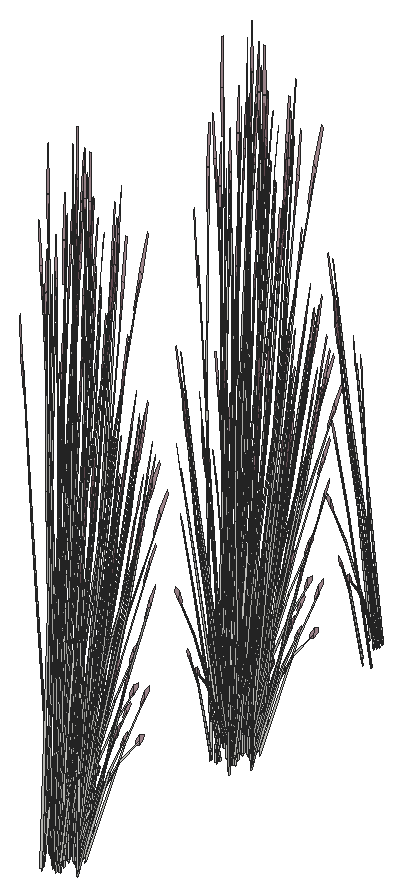
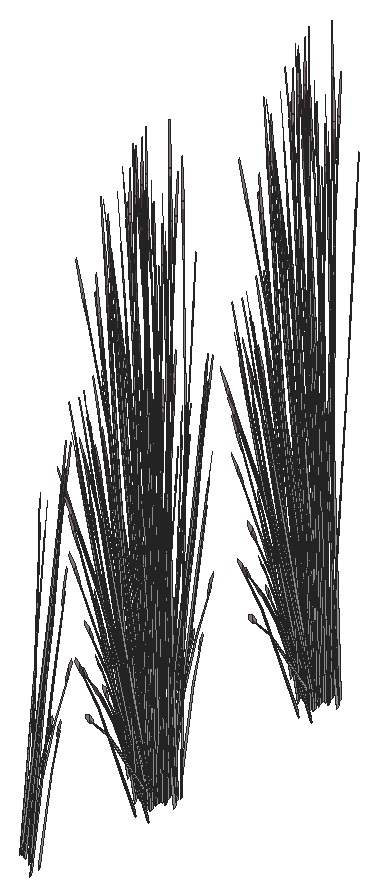
# SketchUp Ruby script. Lengths in inches.
U = 1.inch
M = Sketchup.active_model
def pt(a) = Geom::Point3d.new(a.map { |v| v * U })
def face(e, loops, mat)
  f = e.add_face(loops[0].map { |a| pt(a) })
  loops[1..].each { |l| e.add_face(l.map { |a| pt(a) }).erase! }
  f.material = f.back_material = mat if mat
  f
end
# faces: each face lists its corners as indices into pts; further lists are holes
def faces(e, pts, list, mat = nil) = list.each { |f| face(e, (f[0].is_a?(Array) ? f : [f]).map { |l| l.map { |i| pts[i] } }, mat) }
# xy, xz, yz: faces in a plane at the given z, y or x. An outline is a flat list of corners, or four numbers for a rectangle; further outlines are holes
def ring(l) = l.size == 4 ? [[l[0], l[1]], [l[2], l[1]], [l[2], l[3]], [l[0], l[3]]] : l.each_slice(2).to_a
def flat(e, list, mat, &to3) = list.each { |f| face(e, (f[0].is_a?(Array) ? f : [f]).map { |l| ring(l).map { |u, v| to3.(u, v) } }, mat) }
def xy(e, z, list, mat = nil) = flat(e, list, mat) { |x, y| [x, y, z] }
def xz(e, y, list, mat = nil) = flat(e, list, mat) { |x, z| [x, y, z] }
def yz(e, x, list, mat = nil) = flat(e, list, mat) { |y, z| [x, y, z] }
def lines(e, pts, list) = list.each { |a, b| e.add_line(pt(pts[a]), pt(pts[b])) }
# prism: a flat outline (further loops are holes) pulled along v
def prism(e, loops, v, mat = nil)
  f = face(e, loops, mat); d = Geom::Vector3d.new(v.map { |x| x * U })
  f.pushpull(f.normal.samedirection?(d) ? d.length : -d.length)
end
def box(e, o, s, mat = nil) = prism(e, [[o, [o[0] + s[0], o[1], o[2]], [o[0] + s[0], o[1] + s[1], o[2]], [o[0], o[1] + s[1], o[2]]]], [0, 0, s[2]], mat)
def at(x, y, z, deg = 0) = Geom::Transformation.translation(pt([x, y, z])) * Geom::Transformation.rotation(ORIGIN, Z_AXIS, deg.degrees)
def axes(o, x, y, z) = Geom::Transformation.new([*x, 0, *y, 0, *z, 0, *pt(o).to_a, 1])
def part(name) = M.definitions.add(name)
# library, detail: a bought-in or finely detailed component or shape, given as its bounding box
def library(name, o, s) = part(name).tap { |d| box(d.entities, o, s) }
def detail(e, o, s) = box(e.add_group.entities, o, s)
def put(e, d, t, mat = nil) = e.add_instance(d, t).tap { |i| i.material = mat if mat }
def group(e, t, mat = nil) = e.add_group.tap { |g| g.transformation = t; g.material = mat if mat }.entities
root = M.entities
M.materials.add("LightPink_Translucent").color = [144, 107, 117]
M.materials["LightPink_Translucent"].alpha = 0.75
c1 = part("blade")
p = [[2.15,0.21,22],[0,0.17,0],[0.09,0.45,0],[2.18,0.31,22],[2.29,0.31,22],[0.38,0.45,0],
  [2.48,0.24,33],[2.49,0.24,33],[2.48,0.22,33]]
faces(c1.entities,p,[[0,1,2,3],[4,5,2,3],[6,3,4,7],[8,0,3,6]])
c2 = part("seeds")
p = [[0.3,-0.1,1.38],[-0.01,-0.03,1.59],[-0.01,-0.03,0.03],[0.14,-0.07,-0.07],[0.29,-0.03,3],[0.15,0.01,3.11]]
faces(c2.entities,p,[[0,1,2,3],[1,0,4,5]],"LightPink_Translucent")
c3 = part("blade with seeds")
put(c3.entities,c1,at(0,0,0))
put(c3.entities,c2,axes([2.4,0.25,30.99],[1.5799,-0.05474,1.17369],[-0.12525,1.92788,0.29478],[-0.07173,-0.02425,1.56792]))
put(root,c3,axes([330.71,560.5,1400.21],[0.17124,-0.42022,-0.44739],[0.35581,0.20224,0.21531],[0,-0.09687,1.43643]))
put(root,c3,axes([330.71,582.22,1400.21],[0.17124,-0.42022,-0.44739],[0.35581,0.20224,0.21531],[0,-0.09687,1.43643]))
put(root,c3,axes([331.15,561.85,1400.2],[-0.11516,-0.40207,0],[0.32884,-0.1408,0],[0,0,1.54371]))
put(root,c3,axes([331.15,583.57,1400.2],[-0.11516,-0.40207,0],[0.32884,-0.1408,0],[0,0,1.54371]))
put(root,c3,axes([330.73,562.7,1399.49],[0.05712,-0.02538,1.76342],[0.34359,0.13968,-0.26939],[0.01005,0.15742,0.30037]))
put(root,c3,axes([330.73,584.42,1399.49],[0.05712,-0.02538,1.76342],[0.34359,0.13968,-0.26939],[0.01005,0.15742,0.30037]))
put(root,c3,axes([330.8,562.84,1402.53],[-0.1064,0.35863,-0.35414],[-0.31043,-0.1046,0.4572],[0.02846,0.14439,0.87481]))
put(root,c3,axes([330.8,584.5625,1402.53],[-0.1064,0.35863,-0.35414],[-0.31043,-0.1046,0.4572],[0.02846,0.14439,0.87481]))
put(root,c3,axes([331.61,561.0625,1400.21],[-0.17124,0.42022,-0.44739],[-0.35581,-0.20224,0.21531],[0,0.09687,1.43643]))
put(root,c3,axes([331.61,582.78,1400.21],[-0.17124,0.42022,-0.44739],[-0.35581,-0.20224,0.21531],[0,0.09687,1.43643]))
put(root,c3,axes([331.43,580.4,1402.73],[0.26007,-0.1585,0.0643],[0.12729,0.28902,0.50621],[-0.02512,-0.1274,0.77189]))
put(root,c3,axes([330.58,563.48,1402.72],[0.04474,0.0751,1.74944],[0.36104,0.0295,-0.27667],[0.03631,0.16562,0.14031]))
put(root,c3,axes([330.58,585.2,1402.72],[0.04474,0.0751,1.74944],[0.36104,0.0295,-0.27667],[0.03631,0.16562,0.14031]))
put(root,c3,axes([332.29,560.81,1400.47],[-0.2773,-0.3397,0.17642],[0.27945,-0.32949,0.35086],[-0.03063,0.06937,1.60407]))
put(root,c3,axes([332.29,582.52,1400.47],[-0.2773,-0.3397,0.17642],[0.27945,-0.32949,0.35086],[-0.03063,0.06937,1.60407]))
put(root,c3,axes([331.33,560.61,1400.21],[0,-0.53961,0],[0.44133,0,0],[0,0,1.79456]))
put(root,c3,axes([331.33,582.33,1400.21],[0,-0.53961,0],[0.44133,0,0],[0,0,1.79456]))
put(root,c3,axes([331.34,580.43,1402.73],[0.34777,0.12192,0.48003],[-0.11892,0.40083,0.3958],[-0.0209,-0.15763,0.9933]))
put(root,c3,axes([331.34,599.35,1402.73],[0.34777,0.12192,0.48003],[-0.11892,0.40083,0.3958],[-0.0209,-0.15763,0.9933]))
put(root,c3,axes([330.92,560.71,1400.43],[0.39767,0.22603,0.24065],[-0.19139,0.46966,0.50002],[0,-0.10827,1.60543]))
put(root,c3,axes([330.92,582.43,1400.43],[0.39767,0.22603,0.24065],[-0.19139,0.46966,0.50002],[0,-0.10827,1.60543]))
put(root,c3,axes([331.55,560.82,1400.29],[0,0.53934,-0.05637],[-0.44133,0,0],[0,0.01695,1.79368]))
put(root,c3,axes([331.55,582.54,1400.29],[0,0.53934,-0.05637],[-0.44133,0,0],[0,0.01695,1.79368]))
put(root,c3,axes([330.79,560.39,1400.72],[-0.38326,0.02879,0.44739],[-0.03466,-0.47788,-0.21531],[0.06861,-0.04843,1.43643]))
put(root,c3,axes([330.79,582.11,1400.72],[-0.38326,0.02879,0.44739],[-0.03466,-0.47788,-0.21531],[0.06861,-0.04843,1.43643]))
put(root,c3,axes([330.77,562.47,1403.05],[0.1064,-0.35863,0.35414],[0.31043,0.1046,-0.4572],[0.02846,0.14439,0.87481]))
put(root,c3,axes([330.77,584.18,1403.05],[0.1064,-0.35863,0.35414],[0.31043,0.1046,-0.4572],[0.02846,0.14439,0.87481]))
put(root,c3,axes([330.61,559.57,1400.47],[-0.10196,0.46348,0.17642],[-0.3731,-0.13116,0.35086],[0.06445,-0.00226,1.60407]))
put(root,c3,axes([330.61,581.29,1400.47],[-0.10196,0.46348,0.17642],[-0.3731,-0.13116,0.35086],[0.06445,-0.00226,1.60407]))
put(root,c3,axes([331.34,561.87,1400.29],[0.15345,0.53576,-0.06012],[-0.43845,0.18773,0],[0.00536,0.01871,1.72173]))
put(root,c3,axes([331.34,583.59,1400.29],[0.15345,0.53576,-0.06012],[-0.43845,0.18773,0],[0.00536,0.01871,1.72173]))
put(root,c3,axes([330.43,580.72,1400.375],[-0.22066,-0.46731,0],[0.36918,-0.26061,-0.51607],[0.08408,-0.05936,1.63711]))
put(root,c3,axes([330.84,562.52,1402.98],[0.16845,0.3792,-0.71045],[-0.34676,0.21133,0.08574],[0.03939,0.18322,1.00501]))
put(root,c3,axes([330.84,584.24,1402.98],[0.16845,0.3792,-0.71045],[-0.34676,0.21133,0.08574],[0.03939,0.18322,1.00501]))
put(root,c3,axes([332.61,561.17,1400.2],[-0.44111,-0.00373,-0.04976],[0,-0.52122,0.49943],[-0.01386,0.11865,1.58352]))
put(root,c3,axes([332.61,582.88,1400.2],[-0.44111,-0.00373,-0.04976],[0,-0.52122,0.49943],[-0.01386,0.11865,1.58352]))
put(root,c3,axes([331.74,559.6,1400.47],[-0.37926,0.12378,0.17642],[-0.09365,-0.46065,0.35086],[0.03382,0.06712,1.60407]))
put(root,c3,axes([331.74,581.32,1400.47],[-0.37926,0.12378,0.17642],[-0.09365,-0.46065,0.35086],[0.03382,0.06712,1.60407]))
put(root,c3,axes([331.35,579.59,1400.77],[0.04528,0.27194,1.1486],[-0.25117,-0.15062,0.84392],[0.02703,-0.13924,0.25299]))
put(root,c3,axes([331.35,598.51,1400.77],[0.04528,0.27194,1.1486],[-0.25117,-0.15062,0.84392],[0.02703,-0.13924,0.25299]))
put(root,c3,axes([331.1875,563.75,1403.65],[0.2439,-0.26754,-0.06488],[0.22348,0.29302,-0.29416],[0.01573,0.08303,0.97024]))
put(root,c3,axes([331.1875,585.46,1403.65],[0.2439,-0.26754,-0.06488],[0.22348,0.29302,-0.29416],[0.01573,0.08303,0.97024]))
put(root,c3,axes([331.12,560.27,1400.36],[-0.29264,0.42323,0.45755],[-0.34767,-0.3736,0.17955],[0.07055,-0.04224,1.58856]))
put(root,c3,axes([331.12,581.99,1400.36],[-0.29264,0.42323,0.45755],[-0.34767,-0.3736,0.17955],[0.07055,-0.04224,1.58856]))
put(root,c3,axes([331.62,560.9375,1400.21],[0.24637,0.30123,0],[-0.24637,0.30123,0],[0,0,1.69266]))
put(root,c3,axes([331.62,582.65,1400.21],[0.24637,0.30123,0],[-0.24637,0.30123,0],[0,0,1.69266]))
put(root,c3,axes([331.62,560.58,1400.72],[0.17124,-0.42022,0.44739],[0.35581,0.20224,-0.21531],[0,0.09687,1.43643]))
put(root,c3,axes([331.62,582.3,1400.72],[0.17124,-0.42022,0.44739],[0.35581,0.20224,-0.21531],[0,0.09687,1.43643]))
put(root,c3,axes([331.47,562.04,1400.2],[0.35581,0.20937,0],[-0.17124,0.43505,0],[0,0,1.74954]))
put(root,c3,axes([331.47,583.76,1400.2],[0.35581,0.20937,0],[-0.17124,0.43505,0],[0,0,1.74954]))
put(root,c3,axes([330.96,562.6,1402.68],[0.34695,0.11691,-0.51099],[-0.11892,0.40083,-0.3958],[0.03181,0.16138,0.97773]))
put(root,c3,axes([330.96,584.32,1402.68],[0.34695,0.11691,-0.51099],[-0.11892,0.40083,-0.3958],[0.03181,0.16138,0.97773]))
put(root,c3,axes([330.67,562.62,1403.03],[0.34538,-0.21713,-0.1216],[0.16972,0.38536,-0.67495],[0.04557,0.16239,1.02557]))
put(root,c3,axes([330.67,584.34,1403.03],[0.34538,-0.21713,-0.1216],[0.16972,0.38536,-0.67495],[0.04557,0.16239,1.02557]))
put(root,c3,axes([331.5,560.48,1400.38],[-0.44609,-0.09826,0.49198],[0.09078,-0.55493,0.19306],[0.06519,0.05359,1.70813]))
put(root,c3,axes([331.5,582.2,1400.38],[-0.44609,-0.09826,0.49198],[0.09078,-0.55493,0.19306],[0.06519,0.05359,1.70813]))
put(root,c3,axes([332.43,580.03,1402.71],[-0.03584,0.03562,1.77383],[-0.35118,-0.12018,-0.16761],[-0.01271,-0.15545,0.31391]))
put(root,c3,axes([332.43,598.95,1402.71],[-0.03584,0.03562,1.77383],[-0.35118,-0.12018,-0.16761],[-0.01271,-0.15545,0.31391]))
put(root,c3,axes([332.15,581.0625,1403.03],[-0.3879,-0.02311,-0.1216],[0.0106,-0.43749,-0.67495],[0.02694,-0.1685,1.02557]))
put(root,c3,axes([332.15,599.98,1403.03],[-0.3879,-0.02311,-0.1216],[0.0106,-0.43749,-0.67495],[0.02694,-0.1685,1.02557]))
put(root,c3,axes([332.52,561.24,1400.03],[-0.24637,0.29097,-0.30978],[-0.24637,-0.29097,0.30978],[0,0.09372,1.38974]))
put(root,c3,axes([332.52,582.96,1400.03],[-0.24637,0.29097,-0.30978],[-0.24637,-0.29097,0.30978],[0,0.09372,1.38974]))
put(root,c3,axes([331.8125,561.1875,1400.09],[0.12941,0.42699,-0.69212],[-0.37279,0.15378,-0.18165],[0.0143,0.14459,1.52773]))
put(root,c3,axes([331.8125,582.91,1400.09],[0.12941,0.42699,-0.69212],[-0.37279,0.15378,-0.18165],[0.0143,0.14459,1.52773]))
put(root,c3,axes([331.63,560.73,1400.21],[0.39487,0,0],[0,0.48281,0],[0,0,1.78407]))
put(root,c3,axes([331.63,582.45,1400.21],[0.39487,0,0],[0,0.48281,0],[0,0,1.78407]))
put(root,c3,axes([332,581.13,1403.05],[-0.23881,0.24554,0.35414],[-0.22606,-0.28036,-0.4572],[0.0344,-0.14245,0.87481]))
put(root,c3,axes([331.25,560.2,1400.72],[-0.21202,-0.39143,0.44739],[0.32115,-0.27564,-0.21531],[0.06861,0.04843,1.43643]))
put(root,c3,axes([331.25,581.91,1400.72],[-0.21202,-0.39143,0.44739],[0.32115,-0.27564,-0.21531],[0.06861,0.04843,1.43643]))
put(root,c3,axes([330.86,560.29,1400.67],[-0.04113,-0.53214,-0.29095],[0.42835,-0.03218,-0.50002],[0.07543,-0.07088,1.59708]))
put(root,c3,axes([330.86,582.01,1400.67],[-0.04113,-0.53214,-0.29095],[0.42835,-0.03218,-0.50002],[0.07543,-0.07088,1.59708]))
put(root,c3,axes([331.77,560.68,1400.62],[0.32884,-0.136,0.1448],[0.11516,0.38837,-0.41347],[0,0.08547,1.26744]))
put(root,c3,axes([331.77,582.4,1400.62],[0.32884,-0.136,0.1448],[0.11516,0.38837,-0.41347],[0,0.08547,1.26744]))
put(root,c3,axes([331.89,580.9,1402.68],[-0.25266,-0.31335,-0.51099],[0.2669,-0.27442,-0.3958],[0.03844,-0.15921,0.97773]))
put(root,c3,axes([331.89,599.8125,1402.68],[-0.25266,-0.31335,-0.51099],[0.2669,-0.27442,-0.3958],[0.03844,-0.15921,0.97773]))
put(root,c3,axes([331.65,560.71,1400.67],[0.39748,0.22252,-0.29095],[-0.19139,0.46966,-0.50002],[0.01249,0.11531,1.59708]))
put(root,c3,axes([331.65,582.43,1400.67],[0.39748,0.22252,-0.29095],[-0.19139,0.46966,-0.50002],[0.01249,0.11531,1.59708]))
put(root,c3,axes([330.81,559.11,1400.03],[0.32928,0.11539,-0.30978],[-0.08291,0.40636,0.30978],[0.06638,-0.04686,1.38974]))
put(root,c3,axes([330.81,580.83,1400.03],[0.32928,0.11539,-0.30978],[-0.08291,0.40636,0.30978],[0.06638,-0.04686,1.38974]))
put(root,c3,axes([331.72,580.34,1400.59],[-0.10032,0.0944,1.43002],[-0.30046,-0.16522,-0.30754],[0.05569,-0.20547,0.61141]))
put(root,c3,axes([331.72,599.26,1400.59],[-0.10032,0.0944,1.43002],[-0.30046,-0.16522,-0.30754],[0.05569,-0.20547,0.61141]))
put(root,c3,axes([332.52,560.82,1400.48],[0,-0.46636,0.49651],[0.39487,0,0],[0,0.10622,1.57504]))
put(root,c3,axes([332.52,582.54,1400.48],[0,-0.46636,0.49651],[0.39487,0,0],[0,0.10622,1.57504]))
put(root,c3,axes([332.6875,561.25,1400.02],[0,0.46636,-0.49651],[-0.39487,0,0],[0,0.10622,1.57504]))
put(root,c3,axes([332.6875,582.97,1400.02],[0,0.46636,-0.49651],[-0.39487,0,0],[0,0.10622,1.57504]))
put(root,c3,axes([331.63,562.66,1402.73],[-0.35104,0.10702,0.48003],[-0.06092,-0.41983,0.3958],[0.08256,0.12373,0.9933]))
put(root,c3,axes([331.63,584.38,1402.73],[-0.35104,0.10702,0.48003],[-0.06092,-0.41983,0.3958],[0.08256,0.12373,0.9933]))
put(root,c3,axes([330.73,558.93,1400.02],[0.33032,-0.23318,-0.49651],[0.19744,0.41812,0],[0.07523,-0.05311,1.57504]))
put(root,c3,axes([330.73,580.65,1400.02],[0.33032,-0.23318,-0.49651],[0.19744,0.41812,0],[0.07523,-0.05311,1.57504]))
put(root,c3,axes([331.56,562.75,1402.73],[-0.16041,0.29625,0.0643],[-0.22843,-0.17248,0.50621],[0.07385,0.09498,0.77189]))
put(root,c3,axes([331.56,584.46,1402.73],[-0.16041,0.29625,0.0643],[-0.22843,-0.17248,0.50621],[0.07385,0.09498,0.77189]))
put(root,c3,axes([331.16,561.77,1401.875],[-0.08068,-0.14973,1.71376],[0.3728,-0.12606,0.13857],[0.08426,0.23506,0.73262]))
put(root,c3,axes([331.16,583.49,1401.875],[-0.08068,-0.14973,1.71376],[0.3728,-0.12606,0.13857],[0.08426,0.23506,0.73262]))
put(root,c3,axes([331.39,560.09,1400.62],[0.06809,-0.4162,0.1448],[0.33266,0.07225,-0.41347],[0.06054,0.04274,1.26744]))
put(root,c3,axes([331.39,581.8,1400.62],[0.06809,-0.4162,0.1448],[0.33266,0.07225,-0.41347],[0.06054,0.04274,1.26744]))
put(root,c3,axes([331.87,559.36,1400.48],[-0.33032,-0.23318,0.49651],[0.19744,-0.41812,0],[0.07523,0.05311,1.57504]))
put(root,c3,axes([331.87,581.08,1400.48],[-0.33032,-0.23318,0.49651],[0.19744,-0.41812,0],[0.07523,0.05311,1.57504]))
put(root,c3,axes([331.97,581.04,1402.98],[0.00918,-0.43138,-0.71045],[0.38672,0.02897,0.08574],[0.04081,-0.18275,1.00501]))
put(root,c3,axes([331.97,599.96,1402.98],[0.00918,-0.43138,-0.71045],[0.38672,0.02897,0.08574],[0.04081,-0.18275,1.00501]))
put(root,c3,axes([331.58,561.8,1400.18],[0.37054,-0.15823,-0.19198],[0.1302,0.45581,0.00008],[0.0409,-0.01749,1.73897]))
put(root,c3,axes([331.58,583.52,1400.18],[0.37054,-0.15823,-0.19198],[0.1302,0.45581,0.00008],[0.0409,-0.01749,1.73897]))
put(root,c3,axes([331.52,562.41,1403.05],[-0.05451,-0.37564,0.35414],[0.31161,-0.09919,-0.4572],[0.0837,0.10765,0.87481]))
put(root,c3,axes([331.52,584.125,1403.05],[-0.05451,-0.37564,0.35414],[0.31161,-0.09919,-0.4572],[0.0837,0.10765,0.87481]))
put(root,c3,axes([331.58,560.44,1400.21],[0.21202,0.39143,-0.44739],[-0.32115,0.27564,0.21531],[0.06861,0.04843,1.43643]))
put(root,c3,axes([331.58,582.16,1400.21],[0.21202,0.39143,-0.44739],[-0.32115,0.27564,0.21531],[0.06861,0.04843,1.43643]))
put(root,c3,axes([331.72,560.25,1402.47],[-0.30498,-0.24231,1.38283],[0.32203,-0.37727,0.59665],[0.0984,0.22736,1.33663]))
put(root,c3,axes([331.72,581.96,1402.47],[-0.30498,-0.24231,1.38283],[0.32203,-0.37727,0.59665],[0.0984,0.22736,1.33663]))
put(root,c3,axes([332.13,580.78,1402.53],[0.23881,-0.24554,-0.35414],[0.22606,0.28036,0.4572],[0.0344,-0.14245,0.87481]))
put(root,c3,axes([332.13,599.7,1402.53],[0.23881,-0.24554,-0.35414],[0.22606,0.28036,0.4572],[0.0344,-0.14245,0.87481]))
put(root,c3,axes([331.21,562.93,1402.71],[0.00104,-0.05646,1.77383],[0.30246,-0.2491,-0.16761],[0.10506,0.08891,0.31391]))
put(root,c3,axes([331.21,584.65,1402.71],[0.00104,-0.05646,1.77383],[0.30246,-0.2491,-0.16761],[0.10506,0.08891,0.31391]))
put(root,c3,axes([332.22,580.91,1402.73],[0.29004,0.02173,0.0643],[-0.00795,0.32812,0.50621],[0.03035,-0.12569,0.77189]))
put(root,c3,axes([332.18,562.22,1400.77],[-0.19872,-0.13409,1.1486],[0.2566,-0.13625,0.84392],[0.06921,0.11541,0.25299]))
put(root,c3,axes([332.18,583.9375,1400.77],[-0.19872,-0.13409,1.1486],[0.2566,-0.13625,0.84392],[0.06921,0.11541,0.25299]))
put(root,c3,axes([331.48,562.08,1400.59],[0.00623,-0.15459,1.43002],[0.29764,-0.17268,-0.30754],[0.09188,0.18503,0.61141]))
put(root,c3,axes([331.48,583.79,1400.59],[0.00623,-0.15459,1.43002],[0.29764,-0.17268,-0.30754],[0.09188,0.18503,0.61141]))
put(root,c3,axes([332.51,580.37,1402.72],[-0.00341,-0.09282,1.74944],[-0.28775,-0.26825,-0.27667],[0.04449,-0.16261,0.14031]))
put(root,c3,axes([332.51,599.28,1402.72],[-0.00341,-0.09282,1.74944],[-0.28775,-0.26825,-0.27667],[0.04449,-0.16261,0.14031]))
put(root,c3,axes([331.12,559.88,1400.06],[0.23773,-0.35053,-0.62353],[0.29532,0.31785,-0.16365],[0.09526,-0.08744,1.37633]))
put(root,c3,axes([331.12,581.6,1400.06],[0.23773,-0.35053,-0.62353],[0.29532,0.31785,-0.16365],[0.09526,-0.08744,1.37633]))
put(root,c3,axes([332.125,580.875,1402.73],[0.25132,0.3182,0.48003],[-0.2669,0.27442,0.3958],[0.04636,-0.14929,0.9933]))
put(root,c3,axes([332.17,559.57,1400.03],[0.08291,0.40636,-0.30978],[-0.32928,0.11539,0.30978],[0.06638,0.04686,1.38974]))
put(root,c3,axes([332.17,581.29,1400.03],[0.08291,0.40636,-0.30978],[-0.32928,0.11539,0.30978],[0.06638,0.04686,1.38974]))
put(root,c3,axes([332.78,560.9,1400.375],[0.44133,0,0],[0,0.52122,-0.51607],[0,0.11871,1.63711]))
put(root,c3,axes([332.78,582.62,1400.375],[0.44133,0,0],[0,0.52122,-0.51607],[0,0.11871,1.63711]))
put(root,c3,axes([331.36,560.22,1400.67],[0.35635,-0.30962,-0.29095],[0.23697,0.43749,-0.50002],[0.08792,0.04443,1.59708]))
put(root,c3,axes([331.36,581.94,1400.67],[0.35635,-0.30962,-0.29095],[0.23697,0.43749,-0.50002],[0.08792,0.04443,1.59708]))
put(root,c3,axes([332.22,562.83,1400.67],[-0.22633,-0.01463,1.0506],[0.14947,-0.31064,0.58006],[0.08941,0.11036,0.8241]))
put(root,c3,axes([332.22,584.55,1400.67],[-0.22633,-0.01463,1.0506],[0.14947,-0.31064,0.58006],[0.08941,0.11036,0.8241]))
put(root,c3,axes([332.42,560.17,1403.05],[-0.30722,0.06665,0.35414],[-0.08112,-0.381,-0.4572],[0.08804,-0.10234,0.87481]))
put(root,c3,axes([332.42,581.89,1403.05],[-0.30722,0.06665,0.35414],[-0.08112,-0.381,-0.4572],[0.08804,-0.10234,0.87481]))
put(root,c3,axes([331.53,580.82,1401.875],[-0.06572,0.16029,1.71376],[-0.27569,-0.33172,0.13857],[0.12437,-0.20675,0.73262]))
put(root,c3,axes([331.53,599.74,1401.875],[-0.06572,0.16029,1.71376],[-0.27569,-0.33172,0.13857],[0.12437,-0.20675,0.73262]))
put(root,c3,axes([331.49,562.6,1403.03],[0.21031,-0.39918,-0.1216],[0.30457,0.22997,-0.67495],[0.10587,0.11278,1.02557]))
put(root,c3,axes([331.49,584.32,1403.03],[0.21031,-0.39918,-0.1216],[0.30457,0.22997,-0.67495],[0.10587,0.11278,1.02557]))
put(root,c3,axes([330.46,559.95,1399.59],[-0.3474,0.18671,1.28929],[-0.11057,-0.53572,0.50096],[0.21332,0.00891,1.46642]))
put(root,c3,axes([330.46,581.66,1399.59],[-0.3474,0.18671,1.28929],[-0.11057,-0.53572,0.50096],[0.21332,0.00891,1.46642]))
put(root,c3,axes([332.58,581.92,1403.03],[-0.32648,-0.25715,-0.1216],[0.18809,-0.3724,-0.67495],[0.09224,-0.12945,1.02557]))
put(root,c3,axes([331.74,562.4,1402.68],[0.34827,-0.11086,-0.51099],[0.06092,0.41983,-0.3958],[0.09354,0.12031,0.97773]))
put(root,c3,axes([331.74,584.12,1402.68],[0.34827,-0.11086,-0.51099],[0.06092,0.41983,-0.3958],[0.09354,0.12031,0.97773]))
put(root,c3,axes([332.06,559.12,1400.375],[0.22066,-0.46731,0],[0.36918,0.26061,-0.51607],[0.08408,0.05936,1.63711]))
put(root,c3,axes([332.06,580.84,1400.375],[0.22066,-0.46731,0],[0.36918,0.26061,-0.51607],[0.08408,0.05936,1.63711]))
put(root,c3,axes([332.43,580.63,1399.49],[-0.05283,-0.03674,1.76342],[-0.13569,-0.41045,-0.26939],[0.09154,-0.11138,0.30037]))
put(root,c3,axes([332.14,561.9,1403.05],[-0.20082,-0.29199,0.35414],[0.2293,-0.2764,-0.4572],[0.1165,0.04206,0.87481]))
put(root,c3,axes([332.14,583.62,1403.05],[-0.20082,-0.29199,0.35414],[0.2293,-0.2764,-0.4572],[0.1165,0.04206,0.87481]))
put(root,c3,axes([332.26,559.4,1400.02],[0.33032,0.23318,-0.49651],[-0.19744,0.41812,0],[0.07523,0.05311,1.57504]))
put(root,c3,axes([332.26,581.12,1400.02],[0.33032,0.23318,-0.49651],[-0.19744,0.41812,0],[0.07523,0.05311,1.57504]))
put(root,c3,axes([332.32,562.16,1402.73],[-0.01777,0.35463,0.0643],[-0.26836,-0.00972,0.50621],[0.1028,0.03711,0.77189]))
put(root,c3,axes([332.32,583.88,1402.73],[-0.01777,0.35463,0.0643],[-0.26836,-0.00972,0.50621],[0.1028,0.03711,0.77189]))
put(root,c3,axes([332.24,562.72,1399.49],[0.02571,-0.06733,1.76342],[0.32373,-0.19829,-0.26939],[0.09815,0.10263,0.30037]))
put(root,c3,axes([332.24,584.43,1399.49],[0.02571,-0.06733,1.76342],[0.32373,-0.19829,-0.26939],[0.09815,0.10263,0.30037]))
put(root,c3,axes([332.34,562.05,1402.73],[-0.26024,0.30729,0.48003],[-0.22444,-0.32634,0.3958],[0.1221,0.05668,0.9933]))
put(root,c3,axes([332.34,583.77,1402.73],[-0.26024,0.30729,0.48003],[-0.22444,-0.32634,0.3958],[0.1221,0.05668,0.9933]))
put(root,c3,axes([332.41,581.62,1402.68],[-0.09067,-0.42583,-0.51099],[0.34336,-0.07449,-0.3958],[0.0984,-0.11438,0.97773]))
put(root,c3,axes([333.02,562.1,1401.93],[-0.06755,-0.39203,-0.03492],[0.31928,-0.09013,-0.15832],[0.06667,0.02485,0.52218]))
put(root,c3,axes([333.02,583.81,1401.93],[-0.06755,-0.39203,-0.03492],[0.31928,-0.09013,-0.15832],[0.06667,0.02485,0.52218]))
put(root,c3,axes([332.47,561.08,1403.05],[-0.29332,-0.1301,0.35414],[0.08555,-0.37955,-0.4572],[0.11809,-0.0348,0.87481]))
put(root,c3,axes([332.47,582.8,1403.05],[-0.29332,-0.1301,0.35414],[0.08555,-0.37955,-0.4572],[0.11809,-0.0348,0.87481]))
put(root,c3,axes([331.78,560.29,1400.06],[0.36714,0.07646,-0.62353],[-0.07747,0.47163,-0.16365],[0.10956,0.05715,1.37633]))
put(root,c3,axes([331.78,582.01,1400.06],[0.36714,0.07646,-0.62353],[-0.07747,0.47163,-0.16365],[0.10956,0.05715,1.37633]))
put(root,c3,axes([333.34,560.57,1400.26],[-0.21881,-0.29821,-0.06488],[0.23965,-0.27324,-0.29416],[0.0679,-0.01924,0.97024]))
put(root,c3,axes([333.34,582.29,1400.26],[-0.21881,-0.29821,-0.06488],[0.23965,-0.27324,-0.29416],[0.0679,-0.01924,0.97024]))
put(root,c3,axes([332.84,559.05,1400.77],[-0.11756,0.2374,1.1486],[-0.10105,-0.31895,0.84392],[0.09709,-0.07992,0.25299]))
put(root,c3,axes([332.84,580.77,1400.77],[-0.11756,0.2374,1.1486],[-0.10105,-0.31895,0.84392],[0.09709,-0.07992,0.25299]))
put(root,c3,axes([332.7,560.11,1402.73],[0.2423,0.19613,0.0643],[-0.14107,0.2793,0.50621],[0.07768,-0.0903,0.77189]))
put(root,c3,axes([332.7,581.83,1402.73],[0.2423,0.19613,0.0643],[-0.14107,0.2793,0.50621],[0.07768,-0.0903,0.77189]))
put(root,c3,axes([332.63,560.03,1402.73],[0.08753,0.42921,0.48003],[-0.34336,0.07449,0.3958],[0.1012,-0.10094,0.9933]))
put(root,c3,axes([332.63,581.74,1402.73],[0.08753,0.42921,0.48003],[-0.34336,0.07449,0.3958],[0.1012,-0.10094,0.9933]))
put(root,c3,axes([331.7,561.3,1401.875],[-0.1311,-0.08035,1.71376],[0.27131,-0.33708,0.13857],[0.16909,0.15206,0.73262]))
put(root,c3,axes([331.7,583.02,1401.875],[-0.1311,-0.08035,1.71376],[0.27131,-0.33708,0.13857],[0.16909,0.15206,0.73262]))
put(root,c3,axes([333.38,560.09,1402.71],[-0.0461,-0.00354,1.77383],[-0.19143,-0.37951,-0.16761],[0.07688,-0.12478,0.31391]))
put(root,c3,axes([333.38,581.8125,1402.71],[-0.0461,-0.00354,1.77383],[-0.19143,-0.37951,-0.16761],[0.07688,-0.12478,0.31391]))
put(root,c3,axes([332.67,559.94,1402.53],[0.30722,-0.06665,-0.35414],[0.08112,0.381,0.4572],[0.08804,-0.10234,0.87481]))
put(root,c3,axes([332.67,581.66,1402.53],[0.30722,-0.06665,-0.35414],[0.08112,0.381,0.4572],[0.08804,-0.10234,0.87481]))
put(root,c3,axes([332.42,581.79,1402.98],[0.18436,-0.36797,-0.71045],[0.32306,0.26151,0.08574],[0.11008,-0.13332,1.00501]))
put(root,c3,axes([332.73,561.2,1402.73],[0.12963,0.31798,0.0643],[-0.23638,0.15564,0.50621],[0.1042,-0.03071,0.77189]))
put(root,c3,axes([332.73,582.92,1402.73],[0.12963,0.31798,0.0643],[-0.23638,0.15564,0.50621],[0.1042,-0.03071,0.77189]))
put(root,c3,axes([332.42,562.05,1402.53],[0.20082,0.29199,-0.35414],[-0.2293,0.2764,0.4572],[0.1165,0.04206,0.87481]))
put(root,c3,axes([332.42,583.77,1402.53],[0.20082,0.29199,-0.35414],[-0.2293,0.2764,0.4572],[0.1165,0.04206,0.87481]))
put(root,c3,axes([332.19,562.09,1403.03],[0.0189,-0.47427,-0.1216],[0.35781,0.01296,-0.67495],[0.13781,0.03295,1.02557]))
put(root,c3,axes([332.19,583.8,1403.03],[0.0189,-0.47427,-0.1216],[0.35781,0.01296,-0.67495],[0.13781,0.03295,1.02557]))
put(root,c3,axes([332.59,561.21,1403.03],[-0.17758,-0.42229,-0.1216],[0.31518,-0.20752,-0.67495],[0.13282,-0.05572,1.02557]))
put(root,c3,axes([332.59,582.93,1403.03],[-0.17758,-0.42229,-0.1216],[0.31518,-0.20752,-0.67495],[0.13282,-0.05572,1.02557]))
put(root,c3,axes([332.71,561.09,1402.73],[-0.09971,0.42522,0.48003],[-0.32782,-0.1454,0.3958],[0.12892,-0.02555,0.9933]))
put(root,c3,axes([332.71,582.8,1402.73],[-0.09971,0.42522,0.48003],[-0.32782,-0.1454,0.3958],[0.12892,-0.02555,0.9933]))
put(root,c3,axes([332.5,561.8,1402.72],[0.07571,-0.00789,1.74944],[0.20767,-0.36231,-0.27667],[0.13467,0.04783,0.14031]))
put(root,c3,axes([332.5,583.52,1402.72],[0.07571,-0.00789,1.74944],[0.20767,-0.36231,-0.27667],[0.13467,0.04783,0.14031]))
put(root,c3,axes([332.57,560.85,1402.68],[0.09562,-0.42421,-0.51099],[0.32782,0.1454,-0.3958],[0.13199,-0.0389,0.97773]))
put(root,c3,axes([332.57,582.5625,1402.68],[0.09562,-0.42421,-0.51099],[0.32782,0.1454,-0.3958],[0.13199,-0.0389,0.97773]))
put(root,c3,axes([333.4,561.12,1400.77],[-0.21807,0.07699,1.1486],[0.10265,-0.31819,0.84392],[0.11568,0.02177,0.25299]))
put(root,c3,axes([333.4,582.83,1400.77],[-0.21807,0.07699,1.1486],[0.10265,-0.31819,0.84392],[0.11568,0.02177,0.25299]))
put(root,c3,axes([332.69,559.73,1400.59],[-0.12609,-0.01381,1.43002],[-0.12917,-0.37055,-0.30754],[0.1549,-0.10482,0.61141]))
put(root,c3,axes([332.69,581.45,1400.59],[-0.12609,-0.01381,1.43002],[-0.12917,-0.37055,-0.30754],[0.1549,-0.10482,0.61141]))
put(root,c3,axes([332.78,561.04,1402.53],[0.29332,0.1301,-0.35414],[-0.08555,0.37955,0.4572],[0.11809,-0.0348,0.87481]))
put(root,c3,axes([332.78,582.76,1402.53],[0.29332,0.1301,-0.35414],[-0.08555,0.37955,0.4572],[0.11809,-0.0348,0.87481]))
put(root,c3,axes([332.21,561.86,1402.98],[0.35281,0.01123,-0.71045],[-0.0237,0.47284,0.08574],[0.14947,0.0499,1.00501]))
put(root,c3,axes([332.21,583.57,1402.98],[0.35281,0.01123,-0.71045],[-0.0237,0.47284,0.08574],[0.14947,0.0499,1.00501]))
put(root,c3,axes([332.92,560.97,1399.98],[-0.22732,0.05597,1.41583],[-0.03618,-0.44548,0.08104],[0.15921,-0.06743,0.80566]))
put(root,c3,axes([332.92,582.68,1399.98],[-0.22732,0.05597,1.41583],[-0.03618,-0.44548,0.08104],[0.15921,-0.06743,0.80566]))
put(root,c3,axes([333.17,560.67,1399.49],[-0.01845,-0.0708,1.76342],[0.12793,-0.41416,-0.26939],[0.12905,-0.00596,0.30037]))
put(root,c3,axes([333.17,582.39,1399.49],[-0.01845,-0.0708,1.76342],[0.12793,-0.41416,-0.26939],[0.12905,-0.00596,0.30037]))
put(root,c3,axes([333.3,562.46,1402.71],[-0.03191,-0.04083,1.77383],[0.06981,-0.43764,-0.16761],[0.12571,-0.02796,0.31391]))
put(root,c3,axes([333.3,584.18,1402.71],[-0.03191,-0.04083,1.77383],[0.06981,-0.43764,-0.16761],[0.12571,-0.02796,0.31391]))
put(root,c3,axes([331.98,560.57,1401.875],[-0.14639,0.01056,1.71376],[0.09712,-0.45778,0.13857],[0.20862,0.02831,0.73262]))
put(root,c3,axes([331.98,582.29,1401.875],[-0.14639,0.01056,1.71376],[0.09712,-0.45778,0.13857],[0.20862,0.02831,0.73262]))
put(root,c3,axes([332.51,561,1402.98],[0.31014,-0.20596,-0.71045],[0.17284,0.42397,0.08574],[0.14985,-0.04816,1.00501]))
put(root,c3,axes([332.51,582.72,1402.98],[0.31014,-0.20596,-0.71045],[0.17284,0.42397,0.08574],[0.14985,-0.04816,1.00501]))
put(root,c3,axes([333.55,560.55,1402.72],[0.04898,-0.07104,1.74944],[-0.06269,-0.43574,-0.27667],[0.12289,-0.08262,0.14031]))
put(root,c3,axes([333.55,582.26,1402.72],[0.04898,-0.07104,1.74944],[-0.06269,-0.43574,-0.27667],[0.12289,-0.08262,0.14031]))
put(root,c3,axes([332.99,561.625,1400.59],[-0.085,-0.1147,1.43002],[0.1106,-0.37943,-0.30754],[0.17198,0.0514,0.61141]))
put(root,c3,axes([332.99,583.34,1400.59],[-0.085,-0.1147,1.43002],[0.1106,-0.37943,-0.30754],[0.17198,0.0514,0.61141]))
